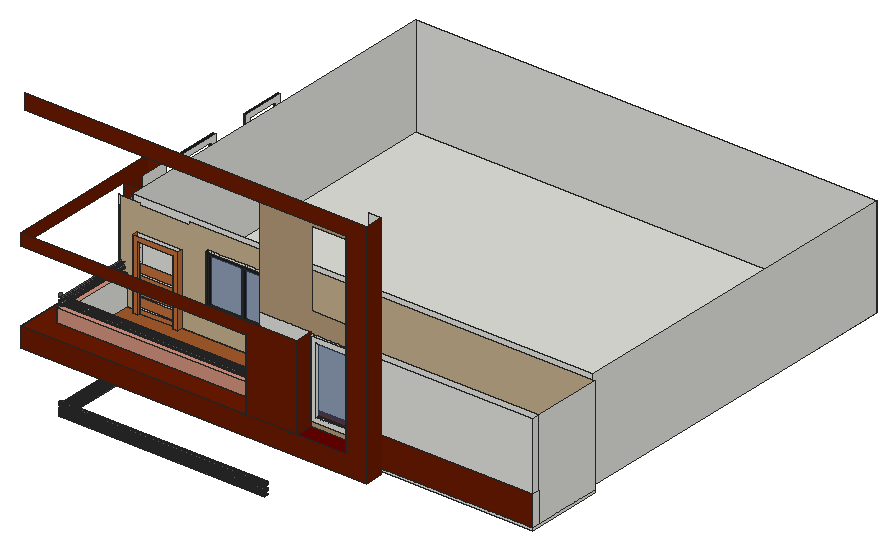
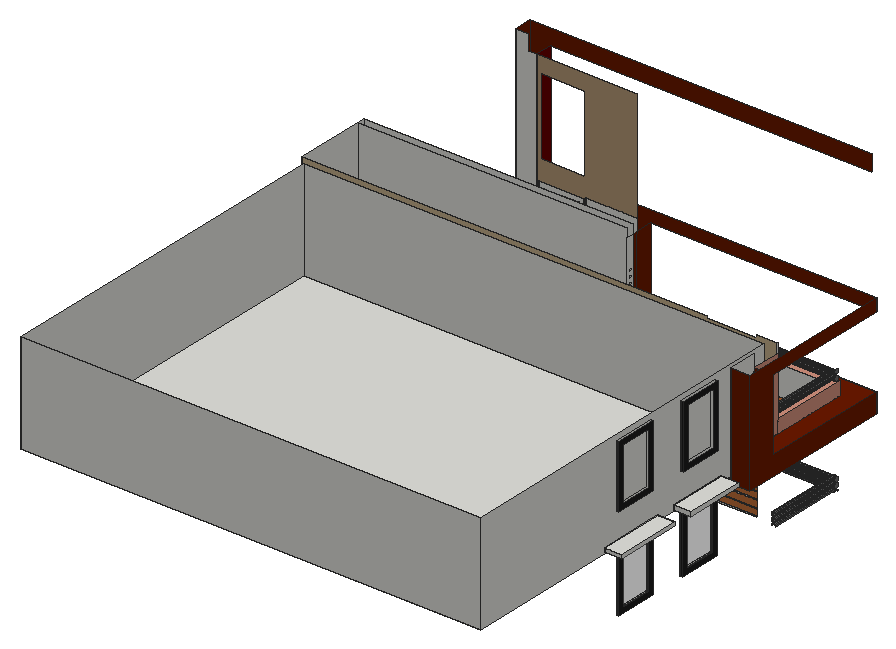
# SketchUp Ruby script. Lengths in inches.
U = 1.inch
M = Sketchup.active_model
def pt(a) = Geom::Point3d.new(a.map { |v| v * U })
def face(e, loops, mat)
  f = e.add_face(loops[0].map { |a| pt(a) })
  loops[1..].each { |l| e.add_face(l.map { |a| pt(a) }).erase! }
  f.material = f.back_material = mat if mat
  f
end
# faces: each face lists its corners as indices into pts; further lists are holes
def faces(e, pts, list, mat = nil) = list.each { |f| face(e, (f[0].is_a?(Array) ? f : [f]).map { |l| l.map { |i| pts[i] } }, mat) }
# xy, xz, yz: faces in a plane at the given z, y or x. An outline is a flat list of corners, or four numbers for a rectangle; further outlines are holes
def ring(l) = l.size == 4 ? [[l[0], l[1]], [l[2], l[1]], [l[2], l[3]], [l[0], l[3]]] : l.each_slice(2).to_a
def flat(e, list, mat, &to3) = list.each { |f| face(e, (f[0].is_a?(Array) ? f : [f]).map { |l| ring(l).map { |u, v| to3.(u, v) } }, mat) }
def xy(e, z, list, mat = nil) = flat(e, list, mat) { |x, y| [x, y, z] }
def xz(e, y, list, mat = nil) = flat(e, list, mat) { |x, z| [x, y, z] }
def yz(e, x, list, mat = nil) = flat(e, list, mat) { |y, z| [x, y, z] }
def lines(e, pts, list) = list.each { |a, b| e.add_line(pt(pts[a]), pt(pts[b])) }
# prism: a flat outline (further loops are holes) pulled along v
def prism(e, loops, v, mat = nil)
  f = face(e, loops, mat); d = Geom::Vector3d.new(v.map { |x| x * U })
  f.pushpull(f.normal.samedirection?(d) ? d.length : -d.length)
end
def box(e, o, s, mat = nil) = prism(e, [[o, [o[0] + s[0], o[1], o[2]], [o[0] + s[0], o[1] + s[1], o[2]], [o[0], o[1] + s[1], o[2]]]], [0, 0, s[2]], mat)
def at(x, y, z, deg = 0) = Geom::Transformation.translation(pt([x, y, z])) * Geom::Transformation.rotation(ORIGIN, Z_AXIS, deg.degrees)
def axes(o, x, y, z) = Geom::Transformation.new([*x, 0, *y, 0, *z, 0, *pt(o).to_a, 1])
def part(name) = M.definitions.add(name)
# library, detail: a bought-in or finely detailed component or shape, given as its bounding box
def library(name, o, s) = part(name).tap { |d| box(d.entities, o, s) }
def detail(e, o, s) = box(e.add_group.entities, o, s)
def put(e, d, t, mat = nil) = e.add_instance(d, t).tap { |i| i.material = mat if mat }
def group(e, t, mat = nil) = e.add_group.tap { |g| g.transformation = t; g.material = mat if mat }.entities
root = M.entities
M.materials.add("[0032_Moccasin]").color = [198, 177, 141]
M.materials.add("[0035_Tan]").color = [181, 154, 120]
M.materials.add("[0134_DimGray]").color = [105, 105, 105]
M.materials.add("[Color A08]").color = [102, 0, 0]
M.materials.add("[Color B02]").color = [209, 145, 125]
M.materials.add("[Color B07]").color = [107, 26, 0]
M.materials.add("[Color M08]").color = [30, 30, 30]
M.materials.add("[Translucent Glass Blue]").color = [61, 91, 145]
M.materials["[Translucent Glass Blue]"].alpha = 0.5
M.materials.add("[Translucent Glass Gray]").color = [128, 128, 128]
M.materials["[Translucent Glass Gray]"].alpha = 0.5
M.materials.add("[Wood Square Tile 01]").color = [164, 91, 44]
M.materials.add("[Wood Veneer 01]").color = [191, 111, 58]
xy(root,546.33,[[31.875,214.36,34.875,265.67],[31.875,309.92,34.875,361.23]],"[Color M08]")
xy(root,552.33,[[31.875,315.92,34.875,355.23]])
xy(root,552.33,[[31.875,220.36,34.875,259.67]],"[Color M08]")
xy(root,576,[[62.21,116.9375,110.21,119.9375]])
xy(root,576,[[62.21,113.9375,110.21,116.9375]],"[Wood Veneer 01]")
xy(root,582,[[56.21,113.9375,116.21,119.9375]],"[Wood Veneer 01]")
xy(root,587,[[144.33,116.9375,184.18,119.9375],[187.18,116.9375,224.02,119.9375]],"[Color M08]")
xy(root,590,[[141.33,116.9375,227.02,119.9375]],"[Color M08]")
xy(root,600.77,[[352.1,17.9375,393.78,20.9375]])
xy(root,606.77,[[346.1,17.9375,399.78,20.9375]])
xy(root,612,[[34.875,26.9375,34.875,119.9375,604.125,119.9375,604.125,35.9375,282.125,35.9375,282.125,26.9375],[282.125,26.9375,604.125,35.9375],[43.875,128.9375,595.125,552.98]])
xy(root,612,[[12.5625,0,400.59,20.9375],[400.59,0,427.625,20.9375],[12.5625,20.9375,12.5625,189.6875,34.875,189.6875,34.875,26.9375,282.125,26.9375,282.125,20.9375]],"[Color B07]")
xy(root,615,[[34.875,26.9375,34.875,119.9375,43.875,119.9375,43.875,35.9375,604.125,35.9375,604.125,26.9375],[56.21,113.9375,62.21,119.9375],[104.21,113.9375,106.03,119.9375],[106.03,113.9375,110.21,119.9375],[62.21,116.9375,104.21,119.9375]])
xy(root,615,[[43.875,35.9375,604.125,35.9375,604.125,119.9375,110.21,119.9375,110.21,113.9375,104.21,113.9375,104.21,116.9375,62.21,116.9375,62.21,113.9375,56.21,113.9375,56.21,119.9375,43.875,119.9375]],"[Wood Square Tile 01]")
xy(root,615.9375,[[31.875,220.36,34.875,259.67],[31.875,315.92,34.875,355.23]],"[Color M08]")
xy(root,621.9375,[[13.875,204.23,13.875,275.92,34.875,275.92,34.875,265.67,31.875,265.67,31.875,214.36,34.875,214.36,34.875,204.23],[31.875,214.36,34.875,265.67],[13.875,299.55,13.875,378.8,34.875,378.8,34.875,361.23,31.875,361.23,31.875,309.92,34.875,309.92,34.875,299.55],[31.875,309.92,34.875,361.23]])
xy(root,626.625,[[13.875,299.55,34.875,378.8]])
xy(root,626.9375,[[13.875,204.23,34.875,275.92]])
xy(root,635.3,[[282.125,0,343.5,20.9375]])
xy(root,635.3,[[343.5,0,402.53,20.9375]],"[Color A08]")
xy(root,635.3,[[12.5625,0,282.125,0,282.125,26.9375,34.875,26.9375,34.875,154.8125,12.5625,154.8125]],"[Color B07]")
xy(root,642.9,[[346.1,17.9375,399.78,20.9375]])
xy(root,648.6875,[[141.33,116.9375,227.02,119.9375]])
xy(root,648.9,[[352.1,17.9375,393.78,20.9375]])
xy(root,651,[[282.125,26.9375,604.125,35.9375]])
xy(root,651,[[34.875,26.9375,282.125,26.9375,282.125,35.9375,43.875,35.9375,43.875,119.9375,34.875,119.9375]],"[Color B02]")
xy(root,651.6875,[[144.33,116.9375,184.18,119.9375],[187.18,116.9375,224.02,119.9375]],"[Color M08]")
xy(root,658.14,[[31.875,213.17,34.875,264.48],[31.875,309.92,34.875,361.23]],"[Color M08]")
xz(root,0,[[12.5625,612,427.625,612,427.625,888,18.22,888,18.22,869.45,402.53,869.45,402.53,635.3,12.5625,635.3],[282.125,635.3,343.5,635.3,343.5,735.99,12.5625,735.99,12.5625,721.21,282.125,721.21]],"[Color B07]")
xz(root,17.9375,[[[346.1,642.9,399.78,734.71],[352.1,648.9,393.78,728.71]]])
xz(root,20.9375,[[282.125,612,400.59,635.3],[400.59,612,427.625,612,427.625,888,413.18,888,413.18,869.45,402.53,869.45,402.53,635.3,400.59,635.3],[282.125,635.3,343.5,735.99],[[346.1,642.9,399.78,734.71],[352.1,648.9,393.78,728.71]]])
xz(root,20.9375,[[[343.5,635.3,402.53,635.3,402.53,869.45,282.125,869.45,282.125,735.99,343.5,735.99],[344.38,758.875,398.07,850.6875],[346.1,642.9,399.78,734.71]]],"[0035_Tan]")
xz(root,20.9375,[[352.1,648.9,393.78,728.71]],"[Translucent Glass Blue]")
xz(root,26.9375,[[34.875,612,282.125,615],[282.125,612,604.125,615],[34.875,615,282.125,635.3],[282.125,651,604.125,732]])
xz(root,26.9375,[[34.875,635.3,282.125,651]],"[Color B02]")
xz(root,26.9375,[[282.125,615,604.125,651]],"[Color B07]")
xz(root,29.17,[[39.57,653.49,40.18,653.57,40.76,653.81,41.25,654.1875,41.625,654.68,41.76,655,37.375,655,37.51,654.68,37.89,654.1875,38.38,653.81,38.95,653.57],[37.375,655,41.76,655,41.86,655.25,41.94,655.87,41.89,656.23,37.24,656.23,37.19,655.87,37.27,655.25],[37.24,656.23,41.89,656.23,41.86,656.48,41.625,657.05,41.25,657.55,40.76,657.92,40.18,658.16,39.57,658.24,38.95,658.16,38.38,657.92,37.89,657.55,37.51,657.05,37.27,656.48]])
xz(root,35.9375,[[43.875,615,282.125,651],[282.125,615,604.125,651],[282.125,651,604.125,732]])
xz(root,113.9375,[[56.21,615,62.21,615,62.21,693,104.21,693,104.21,615,110.21,615,110.21,699,56.21,699]],"[Wood Veneer 01]")
xz(root,116.9375,[[62.21,534.63,110.21,535.94],[62.21,543.7,110.21,545],[62.21,552.76,110.21,554.07],[62.21,561.82,110.21,563.13],[62.21,620.4375,104.21,622.25],
  [62.21,632.5625,104.21,634.38],[62.21,644.6875,104.21,646.5],[62.21,656.8125,104.21,658.63]])
xz(root,116.9375,[[[141.33,648.6875,227.02,709.375],[144.33,651.6875,184.18,706.375],[187.18,651.6875,224.02,706.375]]],"[Color M08]")
xz(root,116.9375,[[62.21,535.94,110.21,543.7],[62.21,545,110.21,552.76],[62.21,554.07,110.21,561.82],[62.21,563.13,110.21,576],[62.21,615,104.21,620.4375],
  [62.21,622.25,104.21,632.5625],[62.21,634.38,104.21,644.6875],[62.21,646.5,104.21,656.8125],[62.21,658.63,104.21,668.9375]],"[Wood Veneer 01]")
xz(root,119.9375,[[34.875,612,35.6,615],[35.6,612,604.125,615],[34.875,615,35.6,651],[35.6,615,43.875,651],[56.21,615,56.21,699,110.21,699,110.21,615,104.21,615,104.21,693,62.21,693,62.21,615],
  [[141.33,648.6875,227.02,709.375],[144.33,651.6875,184.18,706.375],[187.18,651.6875,224.02,706.375]],[34.875,651,35.6,732]])
xz(root,119.9375,[[[43.875,615,56.21,615,56.21,699,110.21,699,110.21,615,604.125,615,604.125,732,119.96,732,119.96,729,59.96,729,59.96,732,35.6,732,35.6,651,43.875,651],[141.33,648.6875,227.02,709.375],[39.57,653.49,38.95,653.57,38.38,653.81,37.89,654.1875,37.51,654.68,37.27,655.25,37.19,655.87,37.27,656.48,37.51,657.05,37.89,657.55,38.38,657.92,38.95,658.16,39.57,658.24,40.18,658.16,40.76,657.92,41.25,657.55,41.625,657.05,41.86,656.48,41.94,655.87,41.86,655.25,41.625,654.68,41.25,654.1875,40.76,653.81,40.18,653.57]]],"[0032_Moccasin]")
xz(root,119.9375,[[144.33,651.6875,184.18,706.375],[187.18,651.6875,224.02,706.375]],"[Translucent Glass Blue]")
xz(root,128.9375,[[43.875,612,595.125,732]])
xz(root,154.8125,[[12.5625,635.3,34.875,721.21]],"[Color B07]")
xz(root,189.6875,[[12.5625,612,34.875,735.99]],"[Color B07]")
xz(root,204.23,[[13.875,621.9375,34.875,626.9375]])
xz(root,213.17,[[31.875,658.14,34.875,733.75]],"[Color M08]")
xz(root,214.36,[[31.875,546.33,34.875,621.9375]],"[Color M08]")
xz(root,220.36,[[31.875,552.33,34.875,615.9375]],"[Color M08]")
xz(root,259.67,[[31.875,552.33,34.875,615.9375]],"[Color M08]")
xz(root,264.48,[[31.875,658.14,34.875,733.75]],"[Color M08]")
xz(root,265.67,[[31.875,546.33,34.875,621.9375]],"[Color M08]")
xz(root,275.92,[[13.875,621.9375,34.875,626.9375]])
xz(root,299.55,[[13.875,621.9375,34.875,626.625]])
xz(root,309.92,[[31.875,546.33,34.875,621.9375],[31.875,658.14,34.875,733.75]],"[Color M08]")
xz(root,315.92,[[31.875,552.33,34.875,615.9375]],"[Color M08]")
xz(root,355.23,[[31.875,552.33,34.875,615.9375]],"[Color M08]")
xz(root,361.23,[[31.875,546.33,34.875,621.9375],[31.875,658.14,34.875,733.75]],"[Color M08]")
xz(root,378.8,[[13.875,621.9375,34.875,626.625]])
xz(root,552.98,[[43.875,612,595.125,732]])
yz(root,12.5625,[[0,612,0,635.3,154.8125,635.3,154.8125,721.21,0,721.21,0,735.99,189.6875,735.99,189.6875,612]],"[Color B07]")
yz(root,13.875,[[204.23,621.9375,275.92,626.9375],[299.55,621.9375,378.8,626.625]])
yz(root,31.875,[[[214.36,546.33,265.67,621.9375],[220.36,552.33,259.67,615.9375]],[[309.92,546.33,361.23,621.9375],[315.92,552.33,355.23,615.9375]],[[213.17,658.14,264.48,733.75],[219.17,664.14,258.48,727.75]],[[309.92,658.14,361.23,733.75],[315.92,664.14,355.23,727.75]]],"[Color M08]")
yz(root,34.875,[[[214.36,546.33,265.67,621.9375],[220.36,552.33,259.67,615.9375]],[[309.92,546.33,361.23,621.9375],[315.92,552.33,355.23,615.9375]],[26.9375,612,119.9375,615],[119.9375,612,189.6875,615],[26.9375,615,119.9375,635.3],
  [119.9375,615,119.9375,635.3,154.8125,635.3,154.8125,735.99,189.6875,735.99,189.6875,615],[204.23,621.9375,207.05,626.9375],[207.05,621.9375,275.92,626.9375],[299.55,621.9375,309.92,626.625],[309.92,621.9375,378.8,626.625],
  [[213.17,658.14,264.48,733.75],[219.17,664.14,258.48,727.75]],[[309.92,658.14,361.23,733.75],[315.92,664.14,355.23,727.75]]])
yz(root,34.875,[[31.46,538.12,30.85,538.2,30.27,538.4375,29.78,538.8125,29.4,539.31,29.17,539.88,29.09,540.49,29.17,541.11,29.4,541.68,29.78,542.17,30.27,542.55,30.85,542.79,31.46,542.87,32.08,542.79,32.65,542.55,33.14,542.17,33.52,541.68,33.76,541.11,33.84,540.49,33.76,539.88,33.52,539.31,33.14,538.8125,32.65,538.4375,32.08,538.2],[31.46,544.87,30.85,544.95,30.27,545.1875,29.78,545.5625,29.4,546.06,29.17,546.63,29.09,547.24,29.17,547.86,29.4,548.43,29.78,548.92,30.27,549.3,30.85,549.54,31.46,549.62,32.08,549.54,32.65,549.3,33.14,548.92,33.52,548.43,33.76,547.86,33.84,547.24,33.76,546.63,33.52,546.06,33.14,545.5625,32.65,545.1875,32.08,544.95],[31.46,653.24,30.85,653.32,30.27,653.5625,29.78,653.9375,29.4,654.43,29.17,655,29.09,655.62,29.17,656.23,29.4,656.81,29.78,657.3,30.27,657.67,30.85,657.91,31.46,657.99,32.08,657.91,32.65,657.67,33.14,657.3,33.52,656.81,33.76,656.23,33.84,655.62,33.76,655,33.52,654.43,33.14,653.9375,32.65,653.5625,32.08,653.32],[31.46,660.62,30.85,660.7,30.27,660.9375,29.78,661.3125,29.4,661.81,29.17,662.38,29.09,662.99,29.17,663.61,29.4,664.18,29.78,664.67,30.27,665.05,30.85,665.29,31.46,665.37,32.08,665.29,32.65,665.05,33.14,664.67,33.52,664.18,33.76,663.61,33.84,662.99,33.76,662.38,33.52,661.81,33.14,661.3125,32.65,660.9375,32.08,660.7]],"[0134_DimGray]")
yz(root,34.875,[[26.9375,635.3,119.9375,651],[119.9375,635.3,154.8125,721.21]],"[Color B02]")
yz(root,34.875,[[220.36,552.33,259.67,615.9375],[315.92,552.33,355.23,615.9375]],"[Translucent Glass Gray]")
yz(root,43.875,[[128.9375,612,552.98,732],[35.9375,615,119.9375,651]])
yz(root,56.21,[[113.9375,615,119.9375,699]],"[Wood Veneer 01]")
yz(root,62.21,[[116.9375,615,119.9375,693]])
yz(root,62.21,[[113.9375,615,116.9375,693]],"[Wood Veneer 01]")
yz(root,104.21,[[116.9375,615,119.9375,693]])
yz(root,104.21,[[113.9375,615,116.9375,693]],"[Wood Veneer 01]")
yz(root,110.21,[[113.9375,615,119.9375,699]],"[Wood Veneer 01]")
yz(root,141.33,[[116.9375,648.6875,119.9375,709.375]],"[Color M08]")
yz(root,144.33,[[116.9375,651.6875,119.9375,706.375]],"[Color M08]")
yz(root,184.18,[[116.9375,651.6875,119.9375,706.375]],"[Color M08]")
yz(root,187.18,[[116.9375,651.6875,119.9375,706.375]],"[Color M08]")
yz(root,224.02,[[116.9375,651.6875,119.9375,706.375]],"[Color M08]")
yz(root,227.02,[[116.9375,648.6875,119.9375,709.375]],"[Color M08]")
yz(root,282.125,[[20.9375,612,26.9375,635.3],[[26.9375,651,35.9375,721.21],[31.46,653.24,32.08,653.32,32.65,653.5625,33.14,653.9375,33.52,654.43,33.76,655,33.84,655.62,33.76,656.23,33.52,656.81,33.14,657.3,32.65,657.67,32.08,657.91,31.46,657.99,30.85,657.91,30.27,657.67,29.78,657.3,29.4,656.81,29.17,656.23,29.09,655.62,29.17,655,29.4,654.43,29.78,653.9375,30.27,653.5625,30.85,653.32],[31.46,660.62,32.08,660.7,32.65,660.9375,33.14,661.3125,33.52,661.81,33.76,662.38,33.84,662.99,33.76,663.61,33.52,664.18,33.14,664.67,32.65,665.05,32.08,665.29,31.46,665.37,30.85,665.29,30.27,665.05,29.78,664.67,29.4,664.18,29.17,663.61,29.09,662.99,29.17,662.38,29.4,661.81,29.78,661.3125,30.27,660.9375,30.85,660.7],[31.46,667.99,32.08,668.07,32.65,668.3125,33.14,668.6875,33.52,669.18,33.76,669.75,33.84,670.37,33.76,670.98,33.52,671.56,33.14,672.05,32.65,672.42,32.08,672.66,31.46,672.74,30.85,672.66,30.27,672.42,29.78,672.05,29.4,671.56,29.17,670.98,29.09,670.37,29.17,669.75,29.4,669.18,29.78,668.6875,30.27,668.3125,30.85,668.07],[31.46,675.37,32.08,675.45,32.65,675.6875,33.14,676.0625,33.52,676.56,33.76,677.13,33.84,677.74,33.76,678.36,33.52,678.93,33.14,679.42,32.65,679.8,32.08,680.04,31.46,680.12,30.85,680.04,30.27,679.8,29.78,679.42,29.4,678.93,29.17,678.36,29.09,677.74,29.17,677.13,29.4,676.56,29.78,676.0625,30.27,675.6875,30.85,675.45],[31.46,682.74,32.08,682.82,32.65,683.0625,33.14,683.4375,33.52,683.93,33.76,684.5,33.84,685.12,33.76,685.73,33.52,686.31,33.14,686.8,32.65,687.17,32.08,687.41,31.46,687.49,30.85,687.41,30.27,687.17,29.78,686.8,29.4,686.31,29.17,685.73,29.09,685.12,29.17,684.5,29.4,683.93,29.78,683.4375,30.27,683.0625,30.85,682.82]]])
yz(root,282.125,[[0,635.3,20.9375,721.21],[20.9375,635.3,26.9375,721.21]],"[Color B07]")
yz(root,343.5,[[0,635.3,20.9375,735.99]],"[Color B07]")
yz(root,346.1,[[17.9375,642.9,20.9375,734.71]])
yz(root,352.1,[[17.9375,648.9,20.9375,728.71]])
yz(root,393.78,[[17.9375,648.9,20.9375,728.71]])
yz(root,399.78,[[17.9375,642.9,20.9375,734.71]])
yz(root,402.53,[[0,635.3,20.9375,869.45]],"[Color A08]")
yz(root,427.625,[[0,612,20.9375,888]],"[Color B07]")
yz(root,595.125,[[128.9375,612,552.98,732]])
yz(root,604.125,[[26.9375,612,119.9375,615],[26.9375,615,35.9375,651],[35.9375,615,119.9375,732],[26.9375,651,35.9375,732]])
p = [[282.125,29.17,534.36],[282.125,29.4,534.93],[34.875,29.4,534.93],[34.875,29.17,534.36],[37.17,29.17,534.36],[41.89,29.17,534.36],
  [282.125,33.52,534.93],[282.125,33.76,534.36],[34.875,33.76,534.36],[34.875,33.52,534.93],[37.23,119.9375,535.07],[37.15,119.9375,534.46],
  [37.15,29.17,534.46],[37.23,29.17,535.07],[41.9,119.9375,534.46],[41.82,119.9375,535.07],[41.82,29.17,535.07],[41.9,29.17,534.46],
  [282.125,29.78,535.42],[34.875,29.78,535.42],[282.125,33.14,535.42],[34.875,33.14,535.42],[37.47,119.9375,535.65],[37.27,29.17,535.17],
  [37.47,29.17,535.65],[41.58,119.9375,535.65],[41.58,29.17,535.65],[41.78,29.17,535.17],[282.125,30.27,535.8],[34.875,30.27,535.8],
  [282.125,32.65,535.8],[34.875,32.65,535.8],[37.85,119.9375,536.14],[37.85,29.17,536.14],[41.21,119.9375,536.14],[41.21,29.17,536.14],
  [282.125,30.85,536.04],[34.875,30.85,536.04],[282.125,32.08,536.04],[34.875,32.08,536.04],[282.125,31.46,536.12],[34.875,31.46,536.12],
  [38.34,119.9375,536.52],[38.34,29.17,536.52],[40.71,119.9375,536.52],[40.71,29.17,536.52],[38.91,119.9375,536.75],[38.91,29.17,536.75],
  [40.14,119.9375,536.75],[40.14,29.17,536.75],[39.53,119.9375,536.84],[39.53,29.17,536.84],[282.125,31.46,538.12],[282.125,30.85,538.2],
  [34.875,30.85,538.2],[34.875,31.46,538.12],[282.125,32.08,538.2],[34.875,32.08,538.2],[282.125,30.27,538.4375],[34.875,30.27,538.4375],
  [282.125,32.65,538.4375],[34.875,32.65,538.4375],[282.125,29.78,538.8125],[34.875,29.78,538.8125],[282.125,33.14,538.8125],[34.875,33.14,538.8125],
  [38.91,119.9375,538.6],[39.53,119.9375,538.52],[39.53,29.17,538.52],[38.91,29.17,538.6],[40.14,119.9375,538.6],[40.14,29.17,538.6],
  [38.34,119.9375,538.84],[38.34,29.17,538.84],[40.71,119.9375,538.84],[40.71,29.17,538.84],[37.85,119.9375,539.22],[37.85,29.17,539.22],
  [41.21,119.9375,539.22],[41.21,29.17,539.22],[282.125,29.4,539.31],[34.875,29.4,539.31],[282.125,33.52,539.31],[34.875,33.52,539.31],
  [37.47,119.9375,539.71],[37.58,29.17,539.57],[37.47,29.17,539.71],[41.58,119.9375,539.71],[41.58,29.17,539.71],[41.47,29.17,539.57],
  [282.125,29.17,539.88],[41.65,29.17,539.88],[37.4,29.17,539.88],[34.875,29.17,539.88],[282.125,33.76,539.88],[34.875,33.76,539.88],
  [37.23,119.9375,540.28],[37.23,29.17,540.28],[41.82,119.9375,540.28],[41.82,29.17,540.28],[282.125,29.09,540.49],[34.875,29.09,540.49],
  [282.125,33.84,540.49],[34.875,33.84,540.49],[37.15,119.9375,540.9],[37.22,29.17,540.38],[37.17,29.17,540.79],[37.15,29.17,540.9],
  [41.9,119.9375,540.9],[41.9,29.17,540.9],[41.89,29.17,540.79],[41.83,29.17,540.38],[282.125,29.17,541.11],[41.875,29.17,541.11],
  [37.18,29.17,541.11],[34.875,29.17,541.11],[282.125,33.76,541.11],[34.875,33.76,541.11],[37.23,119.9375,541.51],[37.23,29.17,541.51],
  [41.82,119.9375,541.51],[41.82,29.17,541.51],[282.125,29.4,541.68],[34.875,29.4,541.68],[282.125,33.52,541.68],[34.875,33.52,541.68],
  [37.47,119.9375,542.09],[37.27,29.17,541.61],[37.47,29.17,542.09],[41.58,119.9375,542.09],[41.58,29.17,542.09],[41.78,29.17,541.61],
  [282.125,29.78,542.17],[34.875,29.78,542.17],[282.125,33.14,542.17],[34.875,33.14,542.17],[37.85,119.9375,542.58],[37.85,29.17,542.58],
  [41.21,119.9375,542.58],[41.21,29.17,542.58],[282.125,30.27,542.55],[34.875,30.27,542.55],[282.125,32.65,542.55],[34.875,32.65,542.55],
  [282.125,30.85,542.79],[34.875,30.85,542.79],[282.125,32.08,542.79],[34.875,32.08,542.79],[38.34,119.9375,542.95],[38.34,29.17,542.95],
  [40.71,119.9375,542.95],[40.71,29.17,542.95],[282.125,31.46,542.87],[34.875,31.46,542.87],[38.91,119.9375,543.19],[38.91,29.17,543.19],
  [40.14,119.9375,543.19],[40.14,29.17,543.19],[39.53,119.9375,543.27],[39.53,29.17,543.27],[38.91,119.9375,544.98],[39.53,119.9375,544.9],
  [39.53,29.17,544.9],[38.91,29.17,544.98],[40.14,119.9375,544.98],[40.14,29.17,544.98],[282.125,30.85,544.95],[282.125,30.27,545.1875],
  [34.875,30.27,545.1875],[34.875,30.85,544.95],[282.125,31.46,544.87],[34.875,31.46,544.87],[282.125,32.08,544.95],[34.875,32.08,544.95],
  [282.125,32.65,545.1875],[34.875,32.65,545.1875],[38.34,119.9375,545.22],[38.34,29.17,545.22],[40.71,119.9375,545.22],[40.71,29.17,545.22],
  [37.85,119.9375,545.59],[37.85,29.17,545.59],[41.21,119.9375,545.59],[41.21,29.17,545.59],[282.125,29.78,545.5625],[34.875,29.78,545.5625],
  [282.125,33.14,545.5625],[34.875,33.14,545.5625],[37.47,119.9375,546.09],[37.58,29.17,545.94],[37.47,29.17,546.09],[41.58,119.9375,546.09],
  [41.58,29.17,546.09],[41.47,29.17,545.94],[282.125,29.4,546.06],[34.875,29.4,546.06],[282.125,33.52,546.06],[34.875,33.52,546.06],
  [282.125,29.17,546.63],[41.81,29.17,546.63],[37.24,29.17,546.63],[34.875,29.17,546.63],[37.23,119.9375,546.66],[37.4,29.17,546.25],
  [37.23,29.17,546.66],[41.82,119.9375,546.66],[41.82,29.17,546.66],[41.65,29.17,546.25],[282.125,33.76,546.63],[34.875,33.76,546.63],
  [282.125,29.09,547.24],[34.875,29.09,547.24],[282.125,33.84,547.24],[34.875,33.84,547.24],[37.15,119.9375,547.27],[37.22,29.17,546.75],
  [37.17,29.17,547.17],[37.15,29.17,547.27],[41.9,119.9375,547.27],[41.9,29.17,547.27],[41.89,29.17,547.17],[41.83,29.17,546.75],
  [282.125,29.17,547.86],[41.82,29.17,547.86],[37.23,29.17,547.86],[34.875,29.17,547.86],[282.125,33.76,547.86],[34.875,33.76,547.86],
  [37.23,119.9375,547.89],[37.18,29.17,547.48],[37.23,29.17,547.89],[41.82,119.9375,547.89],[41.82,29.17,547.89],[41.875,29.17,547.48],
  [282.125,29.4,548.43],[34.875,29.4,548.43],[37.47,119.9375,548.46],[37.27,29.17,547.98],[37.47,29.17,548.46],[41.58,119.9375,548.46],
  [41.58,29.17,548.46],[41.78,29.17,547.98],[282.125,33.52,548.43],[34.875,33.52,548.43],[282.125,29.78,548.92],[34.875,29.78,548.92],
  [282.125,33.14,548.92],[34.875,33.14,548.92],[37.85,119.9375,548.95],[37.85,29.17,548.95],[41.21,119.9375,548.95],[41.21,29.17,548.95],
  [282.125,30.27,549.3],[34.875,30.27,549.3],[282.125,32.65,549.3],[34.875,32.65,549.3],[38.34,119.9375,549.33],[38.34,29.17,549.33],
  [40.71,119.9375,549.33],[40.71,29.17,549.33],[38.91,119.9375,549.57],[38.91,29.17,549.57],[40.14,119.9375,549.57],[40.14,29.17,549.57],
  [282.125,30.85,549.54],[34.875,30.85,549.54],[282.125,32.08,549.54],[34.875,32.08,549.54],[282.125,31.46,549.62],[34.875,31.46,549.62],
  [39.53,119.9375,549.65],[39.53,29.17,549.65],[282.125,31.46,653.24],[282.125,30.85,653.32],[34.875,30.85,653.32],[34.875,31.46,653.24],
  [282.125,32.08,653.32],[34.875,32.08,653.32],[282.125,30.27,653.5625],[34.875,30.27,653.5625],[282.125,32.65,653.5625],[34.875,32.65,653.5625],
  [38.95,119.9375,653.57],[39.57,119.9375,653.49],[39.57,29.17,653.49],[38.95,29.17,653.57],[40.18,119.9375,653.57],[40.18,29.17,653.57],
  [38.38,119.9375,653.81],[38.38,29.17,653.81],[40.76,119.9375,653.81],[40.76,29.17,653.81],[282.125,29.78,653.9375],[34.875,29.78,653.9375],
  [282.125,33.14,653.9375],[34.875,33.14,653.9375],[37.89,119.9375,654.1875],[37.89,29.17,654.1875],[41.25,119.9375,654.1875],[41.25,29.17,654.1875],
  [282.125,29.4,654.43],[34.875,29.4,654.43],[282.125,33.52,654.43],[34.875,33.52,654.43],[37.51,119.9375,654.68],[37.51,29.17,654.68],
  [41.625,119.9375,654.68],[41.625,29.17,654.68],[282.125,29.17,655],[41.76,29.17,655],[37.375,29.17,655],[34.875,29.17,655],
  [282.125,33.76,655],[34.875,33.76,655],[37.27,119.9375,655.25],[37.27,29.17,655.25],[41.86,119.9375,655.25],[41.86,29.17,655.25],
  [282.125,29.09,655.62],[34.875,29.09,655.62],[282.125,33.84,655.62],[34.875,33.84,655.62],[37.19,119.9375,655.87],[37.19,29.17,655.87],
  [41.94,119.9375,655.87],[41.94,29.17,655.87],[282.125,29.17,656.23],[41.89,29.17,656.23],[37.24,29.17,656.23],[34.875,29.17,656.23],
  [282.125,33.76,656.23],[34.875,33.76,656.23],[37.27,119.9375,656.48],[37.27,29.17,656.48],[41.86,119.9375,656.48],[41.86,29.17,656.48],
  [282.125,29.4,656.81],[34.875,29.4,656.81],[282.125,33.52,656.81],[34.875,33.52,656.81],[37.51,119.9375,657.05],[37.51,29.17,657.05],
  [41.625,119.9375,657.05],[41.625,29.17,657.05],[282.125,29.78,657.3],[34.875,29.78,657.3],[282.125,33.14,657.3],[34.875,33.14,657.3],
  [37.89,119.9375,657.55],[37.89,29.17,657.55],[41.25,119.9375,657.55],[41.25,29.17,657.55],[282.125,30.27,657.67],[34.875,30.27,657.67],
  [282.125,32.65,657.67],[34.875,32.65,657.67],[38.38,119.9375,657.92],[38.38,29.17,657.92],[40.76,119.9375,657.92],[40.76,29.17,657.92],
  [282.125,30.85,657.91],[34.875,30.85,657.91],[282.125,32.08,657.91],[34.875,32.08,657.91],[38.95,119.9375,658.16],[38.95,29.17,658.16],
  [40.18,119.9375,658.16],[40.18,29.17,658.16],[282.125,31.46,657.99],[34.875,31.46,657.99],[39.57,119.9375,658.24],[39.57,29.17,658.24],
  [282.125,31.46,660.62],[282.125,30.85,660.7],[34.875,30.85,660.7],[34.875,31.46,660.62],[282.125,32.08,660.7],[34.875,32.08,660.7],
  [38.95,119.9375,660.76],[39.57,119.9375,660.68],[39.57,29.17,660.68],[38.95,29.17,660.76],[40.18,119.9375,660.76],[40.18,29.17,660.76],
  [282.125,30.27,660.9375],[34.875,30.27,660.9375],[282.125,32.65,660.9375],[34.875,32.65,660.9375],[38.38,119.9375,661],[38.38,29.17,661],
  [40.76,119.9375,661],[40.76,29.17,661],[282.125,29.78,661.3125],[34.875,29.78,661.3125],[282.125,33.14,661.3125],[34.875,33.14,661.3125],
  [37.89,119.9375,661.375],[37.89,29.17,661.375],[41.25,119.9375,661.375],[41.25,29.17,661.375],[282.125,29.4,661.81],[34.875,29.4,661.81],
  [282.125,33.52,661.81],[34.875,33.52,661.81],[37.51,119.9375,661.87],[37.51,29.17,661.87],[41.625,119.9375,661.87],[41.625,29.17,661.87],
  [282.125,29.17,662.38],[41.84,29.17,662.38],[37.3,29.17,662.38],[34.875,29.17,662.38],[282.125,33.76,662.38],[34.875,33.76,662.38],
  [37.27,119.9375,662.4375],[37.375,29.17,662.19],[37.27,29.17,662.4375],[41.86,119.9375,662.4375],[41.86,29.17,662.4375],[41.76,29.17,662.19]]
faces(root,p,[[0,1,2,3,4,5],[6,7,8,9],[10,11,12,13],[14,15,16,17],[1,18,19,2],[20,6,9,21],[22,10,13,23,24],[15,25,26,27,16],
  [18,28,29,19],[30,20,21,31],[32,22,24,33],[25,34,35,26],[28,36,37,29],[38,30,31,39],[36,40,41,37],[40,38,39,41],
  [42,32,33,43],[34,44,45,35],[46,42,43,47],[44,48,49,45],[50,46,47,51],[48,50,51,49],[52,53,54,55],[56,52,55,57],
  [53,58,59,54],[60,56,57,61],[58,62,63,59],[64,60,61,65],[66,67,68,69],[67,70,71,68],[72,66,69,73],[70,74,75,71],
  [76,72,73,77],[74,78,79,75],[62,80,81,63],[82,64,65,83],[84,76,77,85,86],[78,87,88,89,79],[80,90,91,92,93,81],[94,82,83,95],
  [96,84,86,92,97],[87,98,99,91,88],[90,100,101,93,92,91],[102,94,95,103],[104,96,97,105,106,107],[98,108,109,110,111,99],[100,112,113,114,115,101],[116,102,103,117],
  [118,104,107,114,119],[108,120,121,113,109],[112,122,123,115,114,113],[124,116,117,125],[126,118,119,127,128],[120,129,130,131,121],[122,132,133,123],[134,124,125,135],
  [136,126,128,137],[129,138,139,130],[132,140,141,133],[142,134,135,143],[140,144,145,141],[146,142,143,147],[148,136,137,149],[138,150,151,139],
  [144,152,153,145],[152,146,147,153],[154,148,149,155],[150,156,157,151],[158,154,155,159],[156,158,159,157],[160,161,162,163],[161,164,165,162],
  [166,167,168,169],[170,166,169,171],[172,170,171,173],[174,172,173,175],[176,160,163,177],[164,178,179,165],[180,176,177,181],[178,182,183,179],
  [167,184,185,168],[186,174,175,187],[188,180,181,189,190],[182,191,192,193,183],[184,194,195,185],[196,186,187,197],[194,198,199,200,201,195],[202,188,190,203,200,204],
  [191,205,206,199,207,192],[208,196,197,209],[198,210,211,201,200,199],[212,208,209,213],[214,202,204,215,216,217],[205,218,219,220,221,206],[210,222,223,224,225,211],[226,212,213,227],
  [228,214,217,229,224,230],[218,231,232,223,233,219],[222,234,235,225,224,223],[236,228,230,237,238],[231,239,240,241,232],[242,226,227,243],[234,244,245,235],[246,242,243,247],
  [248,236,238,249],[239,250,251,240],[244,252,253,245],[254,246,247,255],[256,248,249,257],[250,258,259,251],[260,256,257,261],[258,262,263,259],
  [252,264,265,253],[266,254,255,267],[264,268,269,265],[268,266,267,269],[270,260,261,271],[262,270,271,263],[272,273,274,275],[276,272,275,277],
  [273,278,279,274],[280,276,277,281],[282,283,284,285],[283,286,287,284],[288,282,285,289],[286,290,291,287],[278,292,293,279],[294,280,281,295],
  [296,288,289,297],[290,298,299,291],[292,300,301,293],[302,294,295,303],[304,296,297,305],[298,306,307,299],[300,308,309,310,311,301],[312,302,303,313],
  [314,304,305,310,315],[306,316,317,309,307],[308,318,319,311,310,309],[320,312,313,321],[322,314,315,323],[316,324,325,317],[318,326,327,328,329,319],[330,320,321,331],
  [332,322,323,328,333],[324,334,335,327,325],[326,336,337,329,328,327],[338,330,331,339],[340,332,333,341],[334,342,343,335],[336,344,345,337],[346,338,339,347],
  [348,340,341,349],[342,350,351,343],[344,352,353,345],[354,346,347,355],[356,348,349,357],[350,358,359,351],[352,360,361,353],[362,354,355,363],
  [364,356,357,365],[358,366,367,359],[360,368,369,361],[368,362,363,369],[370,364,365,371],[366,370,371,367],[372,373,374,375],[376,372,375,377],
  [378,379,380,381],[379,382,383,380],[373,384,385,374],[386,376,377,387],[388,378,381,389],[382,390,391,383],[384,392,393,385],[394,386,387,395],
  [396,388,389,397],[390,398,399,391],[392,400,401,393],[402,394,395,403],[404,396,397,405],[398,406,407,399],[400,408,409,410,411,401],[412,402,403,413],
  [414,404,405,415,410,416],[406,417,418,409,419,407]],"[0134_DimGray]")
